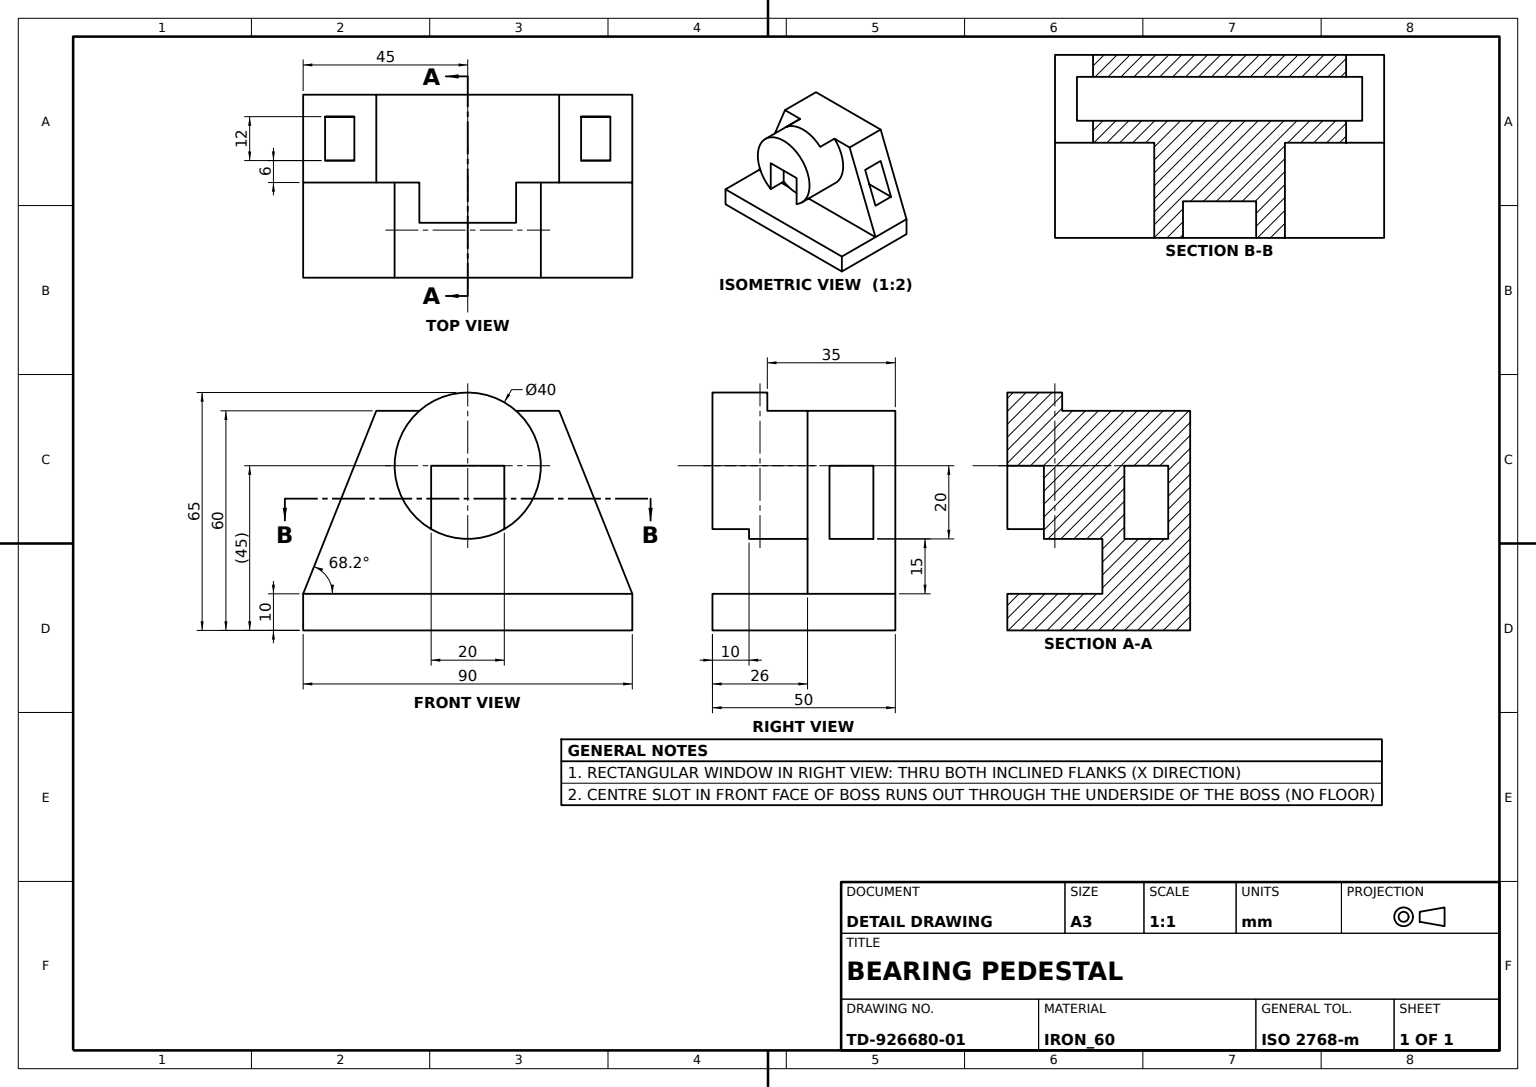
ISO-10303-21;
HEADER;
FILE_DESCRIPTION((''),'2;1');
FILE_NAME('','',(''),(''),'','','');
FILE_SCHEMA(('AUTOMOTIVE_DESIGN'));
ENDSEC;
DATA;
#1=APPLICATION_CONTEXT('');
#2=PRODUCT_CONTEXT('',#1,'mechanical');
#3=PRODUCT('','','',(#2));
#4=PRODUCT_DEFINITION_FORMATION('','',#3);
#5=PRODUCT_DEFINITION_CONTEXT('',#1,'design');
#6=PRODUCT_DEFINITION('','',#4,#5);
#7=PRODUCT_DEFINITION_SHAPE('','',#6);
#8=(LENGTH_UNIT()NAMED_UNIT(*)SI_UNIT(.MILLI.,.METRE.));
#9=(NAMED_UNIT(*)PLANE_ANGLE_UNIT()SI_UNIT($,.RADIAN.));
#10=(NAMED_UNIT(*)SI_UNIT($,.STERADIAN.)SOLID_ANGLE_UNIT());
#11=UNCERTAINTY_MEASURE_WITH_UNIT(LENGTH_MEASURE(0.005),#8,'distance_accuracy_value','');
#12=(GEOMETRIC_REPRESENTATION_CONTEXT(3)GLOBAL_UNCERTAINTY_ASSIGNED_CONTEXT((#11))GLOBAL_UNIT_ASSIGNED_CONTEXT((#8,#9,#10))REPRESENTATION_CONTEXT('',''));
#13=CARTESIAN_POINT('',(25.,-45.,0.));
#14=VERTEX_POINT('',#13);
#15=CARTESIAN_POINT('',(-25.,-45.,0.));
#16=VERTEX_POINT('',#15);
#17=DIRECTION('',(-1.,0.,0.));
#18=VECTOR('',#17,1000.);
#19=LINE('',#13,#18);
#20=EDGE_CURVE('',#14,#16,#19,.T.);
#21=ORIENTED_EDGE('',*,*,#20,.T.);
#22=CARTESIAN_POINT('',(-25.,45.,0.));
#23=VERTEX_POINT('',#22);
#24=DIRECTION('',(0.,-1.,0.));
#25=VECTOR('',#24,1000.);
#26=LINE('',#22,#25);
#27=EDGE_CURVE('',#23,#16,#26,.T.);
#28=ORIENTED_EDGE('',*,*,#27,.F.);
#29=CARTESIAN_POINT('',(25.,45.,0.));
#30=VERTEX_POINT('',#29);
#31=LINE('',#29,#18);
#32=EDGE_CURVE('',#30,#23,#31,.T.);
#33=ORIENTED_EDGE('',*,*,#32,.F.);
#34=LINE('',#29,#25);
#35=EDGE_CURVE('',#30,#14,#34,.T.);
#36=ORIENTED_EDGE('',*,*,#35,.T.);
#37=EDGE_LOOP('',(#21,#28,#33,#36));
#38=FACE_BOUND('',#37,.T.);
#39=DIRECTION('',(0.,0.,-1.));
#40=AXIS2_PLACEMENT_3D('',#29,#39,#17);
#41=PLANE('',#40);
#42=ADVANCED_FACE('',(#38),#41,.T.);
#43=CARTESIAN_POINT('',(-19.,-31.,45.));
#44=VERTEX_POINT('',#43);
#45=CARTESIAN_POINT('',(-19.,-39.,25.));
#46=VERTEX_POINT('',#45);
#47=CARTESIAN_POINT('',(-19.,-25.,60.));
#48=DIRECTION('',(0.,-0.371390676,-0.928476691));
#49=VECTOR('',#48,1000.);
#50=LINE('',#47,#49);
#51=EDGE_CURVE('',#44,#46,#50,.T.);
#52=ORIENTED_EDGE('',*,*,#51,.F.);
#53=CARTESIAN_POINT('',(-7.,-31.,45.));
#54=VERTEX_POINT('',#53);
#55=CARTESIAN_POINT('',(-25.,-31.,45.));
#56=LINE('',#55,#18);
#57=EDGE_CURVE('',#54,#44,#56,.T.);
#58=ORIENTED_EDGE('',*,*,#57,.F.);
#59=CARTESIAN_POINT('',(-7.,-39.,25.));
#60=VERTEX_POINT('',#59);
#61=CARTESIAN_POINT('',(-7.,-25.,60.));
#62=DIRECTION('',(0.,0.371390676,0.928476691));
#63=VECTOR('',#62,1000.);
#64=LINE('',#61,#63);
#65=EDGE_CURVE('',#60,#54,#64,.T.);
#66=ORIENTED_EDGE('',*,*,#65,.F.);
#67=CARTESIAN_POINT('',(-25.,-39.,25.));
#68=DIRECTION('',(1.,0.,0.));
#69=VECTOR('',#68,1000.);
#70=LINE('',#67,#69);
#71=EDGE_CURVE('',#46,#60,#70,.T.);
#72=ORIENTED_EDGE('',*,*,#71,.F.);
#73=EDGE_LOOP('',(#52,#58,#66,#72));
#74=FACE_BOUND('',#73,.T.);
#75=CARTESIAN_POINT('',(-25.,-25.,60.));
#76=VERTEX_POINT('',#75);
#77=CARTESIAN_POINT('',(-25.,-45.,10.));
#78=VERTEX_POINT('',#77);
#79=LINE('',#75,#49);
#80=EDGE_CURVE('',#76,#78,#79,.T.);
#81=ORIENTED_EDGE('',*,*,#80,.T.);
#82=CARTESIAN_POINT('',(-1.,-45.,10.));
#83=VERTEX_POINT('',#82);
#84=LINE('',#77,#69);
#85=EDGE_CURVE('',#78,#83,#84,.T.);
#86=ORIENTED_EDGE('',*,*,#85,.T.);
#87=CARTESIAN_POINT('',(-1.,-25.,60.));
#88=VERTEX_POINT('',#87);
#89=LINE('',#87,#49);
#90=EDGE_CURVE('',#88,#83,#89,.T.);
#91=ORIENTED_EDGE('',*,*,#90,.F.);
#92=LINE('',#75,#69);
#93=EDGE_CURVE('',#76,#88,#92,.T.);
#94=ORIENTED_EDGE('',*,*,#93,.F.);
#95=EDGE_LOOP('',(#81,#86,#91,#94));
#96=FACE_BOUND('',#95,.T.);
#97=DIRECTION('',(0.,-0.928476691,0.371390676));
#98=AXIS2_PLACEMENT_3D('',#75,#97,#48);
#99=PLANE('',#98);
#100=ADVANCED_FACE('',(#74,#96),#99,.T.);
#101=CARTESIAN_POINT('',(10.,13.228757,60.));
#102=VERTEX_POINT('',#101);
#103=CARTESIAN_POINT('',(10.,-13.228757,60.));
#104=VERTEX_POINT('',#103);
#105=CARTESIAN_POINT('',(10.,25.,60.));
#106=LINE('',#105,#25);
#107=EDGE_CURVE('',#102,#104,#106,.T.);
#108=ORIENTED_EDGE('',*,*,#107,.T.);
#109=CARTESIAN_POINT('',(10.,0.,45.));
#110=AXIS2_PLACEMENT_3D('',#109,#68,#39);
#111=CIRCLE('',#110,20.);
#112=EDGE_CURVE('',#102,#104,#111,.T.);
#113=ORIENTED_EDGE('',*,*,#112,.F.);
#114=EDGE_LOOP('',(#108,#113));
#115=FACE_BOUND('',#114,.T.);
#116=CARTESIAN_POINT('',(10.,25.,75.));
#117=AXIS2_PLACEMENT_3D('',#116,#68,#39);
#118=PLANE('',#117);
#119=ADVANCED_FACE('',(#115),#118,.F.);
#120=CARTESIAN_POINT('',(25.,10.,45.));
#121=VERTEX_POINT('',#120);
#122=CARTESIAN_POINT('',(25.,10.,27.679492));
#123=VERTEX_POINT('',#122);
#124=VECTOR('',#39,1000.);
#125=LINE('',#120,#124);
#126=EDGE_CURVE('',#121,#123,#125,.T.);
#127=ORIENTED_EDGE('',*,*,#126,.F.);
#128=CARTESIAN_POINT('',(15.,10.,45.));
#129=VERTEX_POINT('',#128);
#130=LINE('',#120,#18);
#131=EDGE_CURVE('',#129,#121,#130,.F.);
#132=ORIENTED_EDGE('',*,*,#131,.F.);
#133=CARTESIAN_POINT('',(15.,10.,27.679492));
#134=VERTEX_POINT('',#133);
#135=LINE('',#128,#124);
#136=EDGE_CURVE('',#134,#129,#135,.F.);
#137=ORIENTED_EDGE('',*,*,#136,.F.);
#138=LINE('',#122,#18);
#139=EDGE_CURVE('',#123,#134,#138,.T.);
#140=ORIENTED_EDGE('',*,*,#139,.F.);
#141=EDGE_LOOP('',(#127,#132,#137,#140));
#142=FACE_BOUND('',#141,.T.);
#143=DIRECTION('',(0.,1.,0.));
#144=DIRECTION('',(0.,0.,1.));
#145=AXIS2_PLACEMENT_3D('',#120,#143,#144);
#146=PLANE('',#145);
#147=ADVANCED_FACE('',(#142),#146,.F.);
#148=CARTESIAN_POINT('',(15.,-10.,45.));
#149=VERTEX_POINT('',#148);
#150=CARTESIAN_POINT('',(25.,-10.,45.));
#151=VERTEX_POINT('',#150);
#152=LINE('',#150,#18);
#153=EDGE_CURVE('',#149,#151,#152,.F.);
#154=ORIENTED_EDGE('',*,*,#153,.T.);
#155=CARTESIAN_POINT('',(25.,-10.,27.679492));
#156=VERTEX_POINT('',#155);
#157=CARTESIAN_POINT('',(25.,-10.,15.));
#158=VECTOR('',#144,1000.);
#159=LINE('',#157,#158);
#160=EDGE_CURVE('',#156,#151,#159,.T.);
#161=ORIENTED_EDGE('',*,*,#160,.F.);
#162=CARTESIAN_POINT('',(15.,-10.,27.679492));
#163=VERTEX_POINT('',#162);
#164=LINE('',#155,#18);
#165=EDGE_CURVE('',#163,#156,#164,.F.);
#166=ORIENTED_EDGE('',*,*,#165,.F.);
#167=CARTESIAN_POINT('',(15.,-10.,15.));
#168=LINE('',#167,#158);
#169=EDGE_CURVE('',#149,#163,#168,.F.);
#170=ORIENTED_EDGE('',*,*,#169,.F.);
#171=EDGE_LOOP('',(#154,#161,#166,#170));
#172=FACE_BOUND('',#171,.T.);
#173=AXIS2_PLACEMENT_3D('',#157,#24,#39);
#174=PLANE('',#173);
#175=ADVANCED_FACE('',(#172),#174,.F.);
#176=ORIENTED_EDGE('',*,*,#165,.T.);
#177=CARTESIAN_POINT('',(25.,0.,45.));
#178=AXIS2_PLACEMENT_3D('',#177,#68,#143);
#179=CIRCLE('',#178,20.);
#180=EDGE_CURVE('',#123,#156,#179,.T.);
#181=ORIENTED_EDGE('',*,*,#180,.F.);
#182=ORIENTED_EDGE('',*,*,#139,.T.);
#183=CARTESIAN_POINT('',(15.,0.,45.));
#184=AXIS2_PLACEMENT_3D('',#183,#17,#144);
#185=CIRCLE('',#184,20.);
#186=EDGE_CURVE('',#134,#163,#185,.T.);
#187=ORIENTED_EDGE('',*,*,#186,.T.);
#188=EDGE_LOOP('',(#176,#181,#182,#187));
#189=FACE_BOUND('',#188,.T.);
#190=CARTESIAN_POINT('',(-1.,-13.228757,60.));
#191=VERTEX_POINT('',#190);
#192=CARTESIAN_POINT('',(25.,-13.228757,60.));
#193=LINE('',#192,#18);
#194=EDGE_CURVE('',#104,#191,#193,.T.);
#195=ORIENTED_EDGE('',*,*,#194,.T.);
#196=CARTESIAN_POINT('',(-1.,13.228757,60.));
#197=VERTEX_POINT('',#196);
#198=CARTESIAN_POINT('',(-1.,0.,45.));
#199=AXIS2_PLACEMENT_3D('',#198,#68,#143);
#200=CIRCLE('',#199,20.);
#201=EDGE_CURVE('',#191,#197,#200,.T.);
#202=ORIENTED_EDGE('',*,*,#201,.T.);
#203=CARTESIAN_POINT('',(25.,13.228757,60.));
#204=LINE('',#203,#18);
#205=EDGE_CURVE('',#197,#102,#204,.F.);
#206=ORIENTED_EDGE('',*,*,#205,.T.);
#207=ORIENTED_EDGE('',*,*,#112,.T.);
#208=EDGE_LOOP('',(#195,#202,#206,#207));
#209=FACE_BOUND('',#208,.T.);
#210=AXIS2_PLACEMENT_3D('',#177,#17,#144);
#211=CYLINDRICAL_SURFACE('',#210,20.);
#212=ADVANCED_FACE('',(#189,#209),#211,.T.);
#213=CARTESIAN_POINT('',(25.,-45.,10.));
#214=VERTEX_POINT('',#213);
#215=LINE('',#13,#158);
#216=EDGE_CURVE('',#14,#214,#215,.T.);
#217=ORIENTED_EDGE('',*,*,#216,.T.);
#218=LINE('',#213,#18);
#219=EDGE_CURVE('',#214,#83,#218,.T.);
#220=ORIENTED_EDGE('',*,*,#219,.T.);
#221=ORIENTED_EDGE('',*,*,#85,.F.);
#222=LINE('',#15,#158);
#223=EDGE_CURVE('',#16,#78,#222,.T.);
#224=ORIENTED_EDGE('',*,*,#223,.F.);
#225=ORIENTED_EDGE('',*,*,#20,.F.);
#226=EDGE_LOOP('',(#217,#220,#221,#224,#225));
#227=FACE_BOUND('',#226,.T.);
#228=AXIS2_PLACEMENT_3D('',#13,#24,#39);
#229=PLANE('',#228);
#230=ADVANCED_FACE('',(#227),#229,.T.);
#231=CARTESIAN_POINT('',(-1.,25.,60.));
#232=LINE('',#231,#25);
#233=EDGE_CURVE('',#191,#88,#232,.T.);
#234=ORIENTED_EDGE('',*,*,#233,.F.);
#235=ORIENTED_EDGE('',*,*,#194,.F.);
#236=ORIENTED_EDGE('',*,*,#107,.F.);
#237=ORIENTED_EDGE('',*,*,#205,.F.);
#238=VERTEX_POINT('',#231);
#239=EDGE_CURVE('',#238,#197,#232,.T.);
#240=ORIENTED_EDGE('',*,*,#239,.F.);
#241=CARTESIAN_POINT('',(-25.,25.,60.));
#242=VERTEX_POINT('',#241);
#243=LINE('',#241,#69);
#244=EDGE_CURVE('',#242,#238,#243,.T.);
#245=ORIENTED_EDGE('',*,*,#244,.F.);
#246=LINE('',#241,#25);
#247=EDGE_CURVE('',#242,#76,#246,.T.);
#248=ORIENTED_EDGE('',*,*,#247,.T.);
#249=ORIENTED_EDGE('',*,*,#93,.T.);
#250=EDGE_LOOP('',(#234,#235,#236,#237,#240,#245,#248,#249));
#251=FACE_BOUND('',#250,.T.);
#252=AXIS2_PLACEMENT_3D('',#241,#144,#68);
#253=PLANE('',#252);
#254=ADVANCED_FACE('',(#251),#253,.T.);
#255=CARTESIAN_POINT('',(25.,45.,10.));
#256=VERTEX_POINT('',#255);
#257=VECTOR('',#143,1000.);
#258=LINE('',#213,#257);
#259=EDGE_CURVE('',#214,#256,#258,.T.);
#260=ORIENTED_EDGE('',*,*,#259,.F.);
#261=ORIENTED_EDGE('',*,*,#216,.F.);
#262=ORIENTED_EDGE('',*,*,#35,.F.);
#263=LINE('',#255,#124);
#264=EDGE_CURVE('',#256,#30,#263,.T.);
#265=ORIENTED_EDGE('',*,*,#264,.F.);
#266=EDGE_LOOP('',(#260,#261,#262,#265));
#267=FACE_BOUND('',#266,.T.);
#268=CARTESIAN_POINT('',(25.,0.,0.));
#269=AXIS2_PLACEMENT_3D('',#268,#17,#144);
#270=PLANE('',#269);
#271=ADVANCED_FACE('',(#267),#270,.F.);
#272=CARTESIAN_POINT('',(-19.,39.,25.));
#273=VERTEX_POINT('',#272);
#274=CARTESIAN_POINT('',(-19.,-59.,25.));
#275=LINE('',#274,#257);
#276=EDGE_CURVE('',#273,#46,#275,.F.);
#277=ORIENTED_EDGE('',*,*,#276,.F.);
#278=CARTESIAN_POINT('',(-19.,31.,45.));
#279=VERTEX_POINT('',#278);
#280=CARTESIAN_POINT('',(-19.,45.,10.));
#281=DIRECTION('',(0.,-0.371390676,0.928476691));
#282=VECTOR('',#281,1000.);
#283=LINE('',#280,#282);
#284=EDGE_CURVE('',#273,#279,#283,.T.);
#285=ORIENTED_EDGE('',*,*,#284,.T.);
#286=CARTESIAN_POINT('',(-19.,-59.,45.));
#287=LINE('',#286,#257);
#288=EDGE_CURVE('',#279,#44,#287,.F.);
#289=ORIENTED_EDGE('',*,*,#288,.T.);
#290=ORIENTED_EDGE('',*,*,#51,.T.);
#291=EDGE_LOOP('',(#277,#285,#289,#290));
#292=FACE_BOUND('',#291,.T.);
#293=AXIS2_PLACEMENT_3D('',#274,#17,#144);
#294=PLANE('',#293);
#295=ADVANCED_FACE('',(#292),#294,.F.);
#296=ORIENTED_EDGE('',*,*,#180,.T.);
#297=ORIENTED_EDGE('',*,*,#160,.T.);
#298=LINE('',#150,#257);
#299=EDGE_CURVE('',#151,#121,#298,.T.);
#300=ORIENTED_EDGE('',*,*,#299,.T.);
#301=ORIENTED_EDGE('',*,*,#126,.T.);
#302=EDGE_LOOP('',(#296,#297,#300,#301));
#303=FACE_BOUND('',#302,.T.);
#304=AXIS2_PLACEMENT_3D('',#177,#68,#39);
#305=PLANE('',#304);
#306=ADVANCED_FACE('',(#303),#305,.T.);
#307=ORIENTED_EDGE('',*,*,#169,.T.);
#308=ORIENTED_EDGE('',*,*,#186,.F.);
#309=ORIENTED_EDGE('',*,*,#136,.T.);
#310=LINE('',#148,#257);
#311=EDGE_CURVE('',#129,#149,#310,.F.);
#312=ORIENTED_EDGE('',*,*,#311,.T.);
#313=EDGE_LOOP('',(#307,#308,#309,#312));
#314=FACE_BOUND('',#313,.T.);
#315=CARTESIAN_POINT('',(15.,0.,0.));
#316=AXIS2_PLACEMENT_3D('',#315,#17,#144);
#317=PLANE('',#316);
#318=ADVANCED_FACE('',(#314),#317,.F.);
#319=CARTESIAN_POINT('',(-25.,45.,10.));
#320=VERTEX_POINT('',#319);
#321=LINE('',#319,#282);
#322=EDGE_CURVE('',#320,#242,#321,.T.);
#323=ORIENTED_EDGE('',*,*,#322,.T.);
#324=ORIENTED_EDGE('',*,*,#244,.T.);
#325=CARTESIAN_POINT('',(-1.,45.,10.));
#326=VERTEX_POINT('',#325);
#327=LINE('',#325,#282);
#328=EDGE_CURVE('',#326,#238,#327,.T.);
#329=ORIENTED_EDGE('',*,*,#328,.F.);
#330=LINE('',#319,#69);
#331=EDGE_CURVE('',#320,#326,#330,.T.);
#332=ORIENTED_EDGE('',*,*,#331,.F.);
#333=EDGE_LOOP('',(#323,#324,#329,#332));
#334=FACE_BOUND('',#333,.T.);
#335=CARTESIAN_POINT('',(-7.,31.,45.));
#336=VERTEX_POINT('',#335);
#337=CARTESIAN_POINT('',(-25.,31.,45.));
#338=LINE('',#337,#69);
#339=EDGE_CURVE('',#279,#336,#338,.T.);
#340=ORIENTED_EDGE('',*,*,#339,.F.);
#341=ORIENTED_EDGE('',*,*,#284,.F.);
#342=CARTESIAN_POINT('',(-7.,39.,25.));
#343=VERTEX_POINT('',#342);
#344=CARTESIAN_POINT('',(-25.,39.,25.));
#345=LINE('',#344,#18);
#346=EDGE_CURVE('',#343,#273,#345,.T.);
#347=ORIENTED_EDGE('',*,*,#346,.F.);
#348=CARTESIAN_POINT('',(-7.,45.,10.));
#349=DIRECTION('',(0.,0.371390676,-0.928476691));
#350=VECTOR('',#349,1000.);
#351=LINE('',#348,#350);
#352=EDGE_CURVE('',#336,#343,#351,.T.);
#353=ORIENTED_EDGE('',*,*,#352,.F.);
#354=EDGE_LOOP('',(#340,#341,#347,#353));
#355=FACE_BOUND('',#354,.T.);
#356=DIRECTION('',(0.,0.928476691,0.371390676));
#357=AXIS2_PLACEMENT_3D('',#319,#356,#281);
#358=PLANE('',#357);
#359=ADVANCED_FACE('',(#334,#355),#358,.T.);
#360=LINE('',#319,#124);
#361=EDGE_CURVE('',#320,#23,#360,.T.);
#362=ORIENTED_EDGE('',*,*,#361,.T.);
#363=ORIENTED_EDGE('',*,*,#27,.T.);
#364=ORIENTED_EDGE('',*,*,#223,.T.);
#365=ORIENTED_EDGE('',*,*,#80,.F.);
#366=ORIENTED_EDGE('',*,*,#247,.F.);
#367=ORIENTED_EDGE('',*,*,#322,.F.);
#368=EDGE_LOOP('',(#362,#363,#364,#365,#366,#367));
#369=FACE_BOUND('',#368,.T.);
#370=CARTESIAN_POINT('',(-25.,0.,0.));
#371=AXIS2_PLACEMENT_3D('',#370,#68,#39);
#372=PLANE('',#371);
#373=ADVANCED_FACE('',(#369),#372,.F.);
#374=ORIENTED_EDGE('',*,*,#131,.T.);
#375=ORIENTED_EDGE('',*,*,#299,.F.);
#376=ORIENTED_EDGE('',*,*,#153,.F.);
#377=ORIENTED_EDGE('',*,*,#311,.F.);
#378=EDGE_LOOP('',(#374,#375,#376,#377));
#379=FACE_BOUND('',#378,.T.);
#380=AXIS2_PLACEMENT_3D('',#150,#144,#68);
#381=PLANE('',#380);
#382=ADVANCED_FACE('',(#379),#381,.F.);
#383=ORIENTED_EDGE('',*,*,#346,.T.);
#384=ORIENTED_EDGE('',*,*,#276,.T.);
#385=ORIENTED_EDGE('',*,*,#71,.T.);
#386=CARTESIAN_POINT('',(-7.,-59.,25.));
#387=LINE('',#386,#257);
#388=EDGE_CURVE('',#343,#60,#387,.F.);
#389=ORIENTED_EDGE('',*,*,#388,.F.);
#390=EDGE_LOOP('',(#383,#384,#385,#389));
#391=FACE_BOUND('',#390,.T.);
#392=AXIS2_PLACEMENT_3D('',#386,#39,#17);
#393=PLANE('',#392);
#394=ADVANCED_FACE('',(#391),#393,.F.);
#395=ORIENTED_EDGE('',*,*,#288,.F.);
#396=ORIENTED_EDGE('',*,*,#339,.T.);
#397=CARTESIAN_POINT('',(-7.,-59.,45.));
#398=LINE('',#397,#257);
#399=EDGE_CURVE('',#336,#54,#398,.F.);
#400=ORIENTED_EDGE('',*,*,#399,.T.);
#401=ORIENTED_EDGE('',*,*,#57,.T.);
#402=EDGE_LOOP('',(#395,#396,#400,#401));
#403=FACE_BOUND('',#402,.T.);
#404=AXIS2_PLACEMENT_3D('',#286,#144,#68);
#405=PLANE('',#404);
#406=ADVANCED_FACE('',(#403),#405,.F.);
#407=ORIENTED_EDGE('',*,*,#239,.T.);
#408=ORIENTED_EDGE('',*,*,#201,.F.);
#409=ORIENTED_EDGE('',*,*,#233,.T.);
#410=ORIENTED_EDGE('',*,*,#90,.T.);
#411=LINE('',#82,#257);
#412=EDGE_CURVE('',#83,#326,#411,.T.);
#413=ORIENTED_EDGE('',*,*,#412,.T.);
#414=ORIENTED_EDGE('',*,*,#328,.T.);
#415=EDGE_LOOP('',(#407,#408,#409,#410,#413,#414));
#416=FACE_BOUND('',#415,.T.);
#417=CARTESIAN_POINT('',(-1.,0.,0.));
#418=AXIS2_PLACEMENT_3D('',#417,#68,#39);
#419=PLANE('',#418);
#420=ADVANCED_FACE('',(#416),#419,.T.);
#421=ORIENTED_EDGE('',*,*,#219,.F.);
#422=ORIENTED_EDGE('',*,*,#259,.T.);
#423=LINE('',#255,#18);
#424=EDGE_CURVE('',#256,#326,#423,.T.);
#425=ORIENTED_EDGE('',*,*,#424,.T.);
#426=ORIENTED_EDGE('',*,*,#412,.F.);
#427=EDGE_LOOP('',(#421,#422,#425,#426));
#428=FACE_BOUND('',#427,.T.);
#429=AXIS2_PLACEMENT_3D('',#213,#144,#68);
#430=PLANE('',#429);
#431=ADVANCED_FACE('',(#428),#430,.T.);
#432=ORIENTED_EDGE('',*,*,#388,.T.);
#433=ORIENTED_EDGE('',*,*,#65,.T.);
#434=ORIENTED_EDGE('',*,*,#399,.F.);
#435=ORIENTED_EDGE('',*,*,#352,.T.);
#436=EDGE_LOOP('',(#432,#433,#434,#435));
#437=FACE_BOUND('',#436,.T.);
#438=AXIS2_PLACEMENT_3D('',#397,#68,#39);
#439=PLANE('',#438);
#440=ADVANCED_FACE('',(#437),#439,.F.);
#441=ORIENTED_EDGE('',*,*,#264,.T.);
#442=ORIENTED_EDGE('',*,*,#32,.T.);
#443=ORIENTED_EDGE('',*,*,#361,.F.);
#444=ORIENTED_EDGE('',*,*,#331,.T.);
#445=ORIENTED_EDGE('',*,*,#424,.F.);
#446=EDGE_LOOP('',(#441,#442,#443,#444,#445));
#447=FACE_BOUND('',#446,.T.);
#448=AXIS2_PLACEMENT_3D('',#255,#143,#144);
#449=PLANE('',#448);
#450=ADVANCED_FACE('',(#447),#449,.T.);
#451=CLOSED_SHELL('',(#42,#100,#119,#147,#175,#212,#230,#254,#271,#295,#306,#318,#359,#373,#382,#394,#406,#420,#431,#440,#450));
#452=MANIFOLD_SOLID_BREP('',#451);
#453=ADVANCED_BREP_SHAPE_REPRESENTATION('',(#452),#12);
#454=SHAPE_DEFINITION_REPRESENTATION(#7,#453);
ENDSEC;
END-ISO-10303-21;
